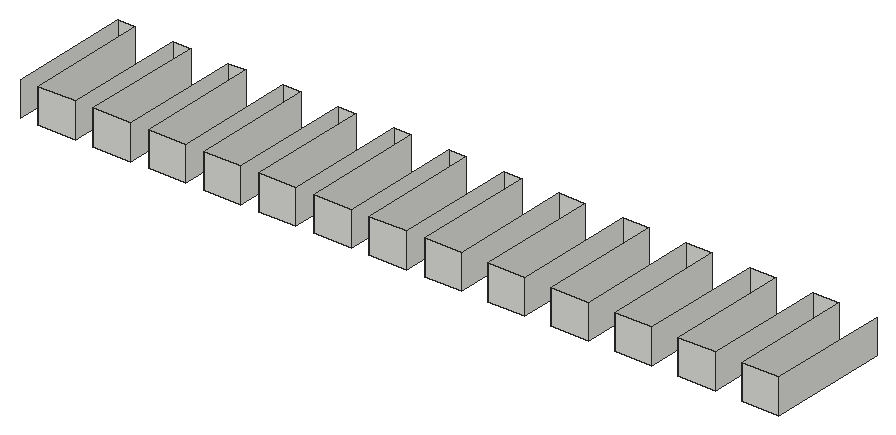
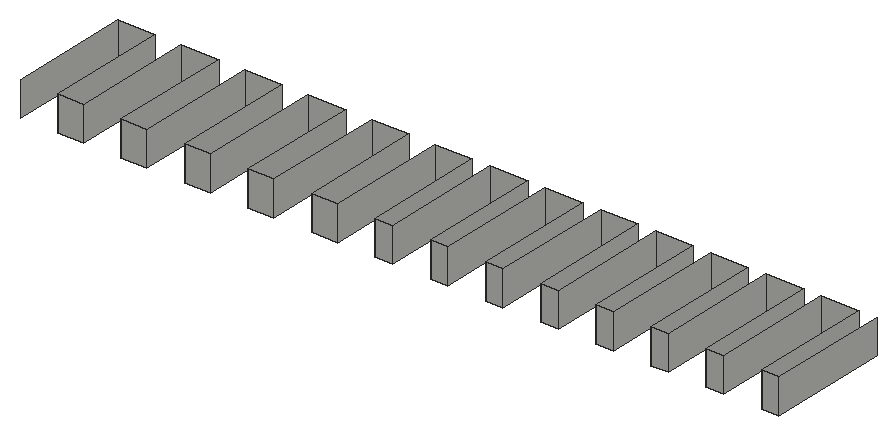
# SketchUp Ruby script. Lengths in inches.
U = 1.inch
M = Sketchup.active_model
def pt(a) = Geom::Point3d.new(a.map { |v| v * U })
def face(e, loops, mat)
  f = e.add_face(loops[0].map { |a| pt(a) })
  loops[1..].each { |l| e.add_face(l.map { |a| pt(a) }).erase! }
  f.material = f.back_material = mat if mat
  f
end
# faces: each face lists its corners as indices into pts; further lists are holes
def faces(e, pts, list, mat = nil) = list.each { |f| face(e, (f[0].is_a?(Array) ? f : [f]).map { |l| l.map { |i| pts[i] } }, mat) }
# xy, xz, yz: faces in a plane at the given z, y or x. An outline is a flat list of corners, or four numbers for a rectangle; further outlines are holes
def ring(l) = l.size == 4 ? [[l[0], l[1]], [l[2], l[1]], [l[2], l[3]], [l[0], l[3]]] : l.each_slice(2).to_a
def flat(e, list, mat, &to3) = list.each { |f| face(e, (f[0].is_a?(Array) ? f : [f]).map { |l| ring(l).map { |u, v| to3.(u, v) } }, mat) }
def xy(e, z, list, mat = nil) = flat(e, list, mat) { |x, y| [x, y, z] }
def xz(e, y, list, mat = nil) = flat(e, list, mat) { |x, z| [x, y, z] }
def yz(e, x, list, mat = nil) = flat(e, list, mat) { |y, z| [x, y, z] }
def lines(e, pts, list) = list.each { |a, b| e.add_line(pt(pts[a]), pt(pts[b])) }
# prism: a flat outline (further loops are holes) pulled along v
def prism(e, loops, v, mat = nil)
  f = face(e, loops, mat); d = Geom::Vector3d.new(v.map { |x| x * U })
  f.pushpull(f.normal.samedirection?(d) ? d.length : -d.length)
end
def box(e, o, s, mat = nil) = prism(e, [[o, [o[0] + s[0], o[1], o[2]], [o[0] + s[0], o[1] + s[1], o[2]], [o[0], o[1] + s[1], o[2]]]], [0, 0, s[2]], mat)
def at(x, y, z, deg = 0) = Geom::Transformation.translation(pt([x, y, z])) * Geom::Transformation.rotation(ORIGIN, Z_AXIS, deg.degrees)
def axes(o, x, y, z) = Geom::Transformation.new([*x, 0, *y, 0, *z, 0, *pt(o).to_a, 1])
def part(name) = M.definitions.add(name)
# library, detail: a bought-in or finely detailed component or shape, given as its bounding box
def library(name, o, s) = part(name).tap { |d| box(d.entities, o, s) }
def detail(e, o, s) = box(e.add_group.entities, o, s)
def put(e, d, t, mat = nil) = e.add_instance(d, t).tap { |i| i.material = mat if mat }
def group(e, t, mat = nil) = e.add_group.tap { |g| g.transformation = t; g.material = mat if mat }.entities
root = M.entities
xz(root,179.27,[[775.09,0,776.79,1.5625],[777.59,0,779.29,1.5625],[780.09,0,781.79,1.5625],[782.59,0,784.29,1.5625],[785.09,0,786.79,1.5625],
  [787.59,0,789.29,1.5625],[790.09,0,791.79,1.5625],[792.59,0,794.29,1.5625],[795.47,0,797.16,1.5625],[798.34,0,800.04,1.5625],
  [801.22,0,802.91,1.5625],[804.09,0,805.79,1.5625],[806.97,0,808.66,1.5625]])
xz(root,184.77,[[774.29,0,775.09,1.5625],[776.79,0,777.59,1.5625],[779.29,0,780.09,1.5625],[781.79,0,782.59,1.5625],[784.29,0,785.09,1.5625],
  [786.79,0,787.59,1.5625],[789.29,0,790.09,1.5625],[791.79,0,792.59,1.5625],[794.29,0,795.47,1.5625],[797.16,0,798.34,1.5625],
  [800.04,0,801.22,1.5625],[802.91,0,804.09,1.5625],[805.79,0,806.97,1.5625]])
yz(root,774.29,[[179.27,0,184.77,1.5625]])
yz(root,775.09,[[179.27,0,184.77,1.5625]])
yz(root,776.79,[[179.27,0,184.77,1.5625]])
yz(root,777.59,[[179.27,0,184.77,1.5625]])
yz(root,779.29,[[179.27,0,184.77,1.5625]])
yz(root,780.09,[[179.27,0,184.77,1.5625]])
yz(root,781.79,[[179.27,0,184.77,1.5625]])
yz(root,782.59,[[179.27,0,184.77,1.5625]])
yz(root,784.29,[[179.27,0,184.77,1.5625]])
yz(root,785.09,[[179.27,0,184.77,1.5625]])
yz(root,786.79,[[179.27,0,184.77,1.5625]])
yz(root,787.59,[[179.27,0,184.77,1.5625]])
yz(root,789.29,[[179.27,0,184.77,1.5625]])
yz(root,790.09,[[179.27,0,184.77,1.5625]])
yz(root,791.79,[[179.27,0,184.77,1.5625]])
yz(root,792.59,[[179.27,0,184.77,1.5625]])
yz(root,794.29,[[179.27,0,184.77,1.5625]])
yz(root,795.47,[[179.27,0,184.77,1.5625]])
yz(root,797.16,[[179.27,0,184.77,1.5625]])
yz(root,798.34,[[179.27,0,184.77,1.5625]])
yz(root,800.04,[[179.27,0,184.77,1.5625]])
yz(root,801.22,[[179.27,0,184.77,1.5625]])
yz(root,802.91,[[179.27,0,184.77,1.5625]])
yz(root,804.09,[[179.27,0,184.77,1.5625]])
yz(root,805.79,[[179.27,0,184.77,1.5625]])
yz(root,806.97,[[179.27,0,184.77,1.5625]])
yz(root,808.66,[[179.27,0,184.77,1.5625]])
